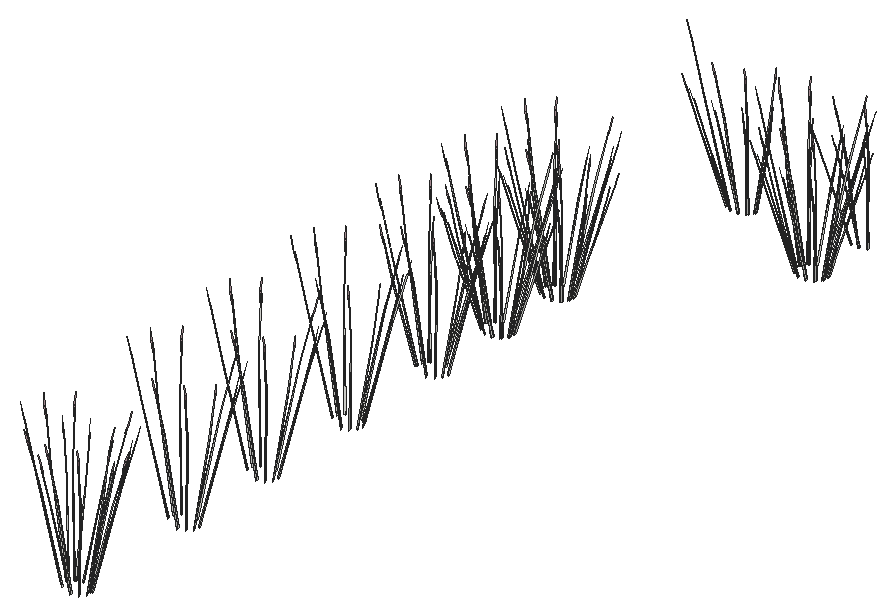
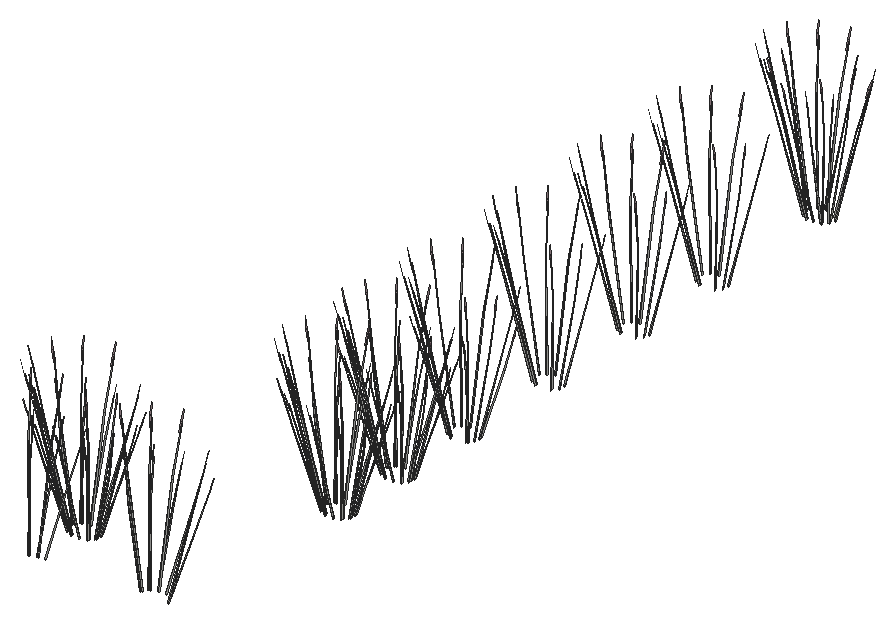
# SketchUp Ruby script. Lengths in inches.
U = 1.inch
M = Sketchup.active_model
def pt(a) = Geom::Point3d.new(a.map { |v| v * U })
def face(e, loops, mat)
  f = e.add_face(loops[0].map { |a| pt(a) })
  loops[1..].each { |l| e.add_face(l.map { |a| pt(a) }).erase! }
  f.material = f.back_material = mat if mat
  f
end
# faces: each face lists its corners as indices into pts; further lists are holes
def faces(e, pts, list, mat = nil) = list.each { |f| face(e, (f[0].is_a?(Array) ? f : [f]).map { |l| l.map { |i| pts[i] } }, mat) }
# xy, xz, yz: faces in a plane at the given z, y or x. An outline is a flat list of corners, or four numbers for a rectangle; further outlines are holes
def ring(l) = l.size == 4 ? [[l[0], l[1]], [l[2], l[1]], [l[2], l[3]], [l[0], l[3]]] : l.each_slice(2).to_a
def flat(e, list, mat, &to3) = list.each { |f| face(e, (f[0].is_a?(Array) ? f : [f]).map { |l| ring(l).map { |u, v| to3.(u, v) } }, mat) }
def xy(e, z, list, mat = nil) = flat(e, list, mat) { |x, y| [x, y, z] }
def xz(e, y, list, mat = nil) = flat(e, list, mat) { |x, z| [x, y, z] }
def yz(e, x, list, mat = nil) = flat(e, list, mat) { |y, z| [x, y, z] }
def lines(e, pts, list) = list.each { |a, b| e.add_line(pt(pts[a]), pt(pts[b])) }
# prism: a flat outline (further loops are holes) pulled along v
def prism(e, loops, v, mat = nil)
  f = face(e, loops, mat); d = Geom::Vector3d.new(v.map { |x| x * U })
  f.pushpull(f.normal.samedirection?(d) ? d.length : -d.length)
end
def box(e, o, s, mat = nil) = prism(e, [[o, [o[0] + s[0], o[1], o[2]], [o[0] + s[0], o[1] + s[1], o[2]], [o[0], o[1] + s[1], o[2]]]], [0, 0, s[2]], mat)
def at(x, y, z, deg = 0) = Geom::Transformation.translation(pt([x, y, z])) * Geom::Transformation.rotation(ORIGIN, Z_AXIS, deg.degrees)
def axes(o, x, y, z) = Geom::Transformation.new([*x, 0, *y, 0, *z, 0, *pt(o).to_a, 1])
def part(name) = M.definitions.add(name)
# library, detail: a bought-in or finely detailed component or shape, given as its bounding box
def library(name, o, s) = part(name).tap { |d| box(d.entities, o, s) }
def detail(e, o, s) = box(e.add_group.entities, o, s)
def put(e, d, t, mat = nil) = e.add_instance(d, t).tap { |i| i.material = mat if mat }
def group(e, t, mat = nil) = e.add_group.tap { |g| g.transformation = t; g.material = mat if mat }.entities
root = M.entities
M.materials.add("LightPink_Translucent").color = [144, 107, 117]
M.materials["LightPink_Translucent"].alpha = 0.75
c1 = part("blade")
p = [[2.15,0.21,22],[0,0.17,0],[0.09,0.45,0],[2.18,0.31,22],[2.29,0.31,22],[0.38,0.45,0],
  [2.48,0.24,33],[2.49,0.24,33],[2.48,0.22,33]]
faces(c1.entities,p,[[0,1,2,3],[4,5,2,3],[6,3,4,7],[8,0,3,6]])
c2 = part("seeds")
p = [[0.3,-0.1,1.38],[-0.01,-0.03,1.59],[-0.01,-0.03,0.03],[0.14,-0.07,-0.07],[0.29,-0.03,3],[0.15,0.01,3.11]]
faces(c2.entities,p,[[0,1,2,3],[1,0,4,5]],"LightPink_Translucent")
c3 = part("blade with seeds")
put(c3.entities,c1,at(0,0,0))
put(c3.entities,c2,axes([2.4,0.25,30.99],[1.5799,-0.05474,1.17369],[-0.12525,1.92788,0.29478],[-0.07173,-0.02425,1.56792]))
put(root,c3,axes([672.23,166.16,513.93],[0.64106,0.14927,0.39842],[-0.21921,0.49074,0.32852],[-0.03852,-0.19299,0.82444]))
put(root,c3,axes([672.22,166.52,514.19],[-0.19614,0.43908,0.29394],[-0.57222,-0.12807,-0.37948],[-0.05247,-0.17678,0.72609]))
put(root,c3,axes([673.68,166.71,513.93],[0.46327,0.38957,0.39842],[-0.49199,0.33598,0.32852],[0.08546,-0.18277,0.82444]))
put(root,c3,axes([674.61,167.77,513.93],[0.16135,0.52549,0.39842],[-0.63294,0.0912,0.32852],[0.18654,-0.12359,0.82444]))
put(root,c3,axes([669.7,167.22,514.19],[0.37017,0.35748,0.29394],[-0.42268,0.3384,-0.37948],[-0.21476,-0.05149,0.72609]))
put(root,c3,axes([674.31,169.0625,514.19],[-0.54068,-0.15928,0.29394],[0.1577,-0.46469,-0.37948],[0.21769,-0.04261,0.72609]))
put(root,c3,axes([668.65,168.21,513.93],[0.18381,-0.5206,0.39842],[0.60429,0.17802,0.32852],[-0.23764,0.03129,0.82444]))
put(root,c3,axes([674.75,169.07,513.93],[-0.18381,0.5206,0.39842],[-0.60429,-0.17802,0.32852],[0.23764,-0.03129,0.82444]))
put(root,c3,axes([673.7,170.07,514.19],[-0.37017,-0.35748,0.29394],[0.42268,-0.3384,-0.37948],[0.21476,0.05149,0.72609]))
put(root,c3,axes([668.8,169.51,513.93],[-0.16135,-0.52549,0.39842],[0.63294,-0.0912,0.32852],[-0.18654,0.12359,0.82444]))
put(root,c3,axes([669.18,169.34,514.19],[0.56631,-0.0816,0.29394],[0.14954,0.46647,-0.37948],[-0.16229,0.12529,0.72609]))
put(root,c3,axes([674.08,170.25,513.93],[-0.47971,0.37622,0.39842],[-0.41372,-0.39954,0.32852],[0.22506,0.0694,0.82444]))
put(root,c3,axes([669.95,170.26,514.19],[0.4402,-0.30062,0.29394],[0.41671,0.34326,-0.37948],[-0.0634,0.1744,0.72609]))
put(root,c3,axes([669.72,170.57,513.93],[-0.46327,-0.38957,0.39842],[0.49199,-0.33598,0.32852],[-0.08546,0.18277,0.82444]))
put(root,c3,axes([671.18,170.76,514.19],[0.19614,-0.43908,0.29394],[0.57222,0.12807,-0.37948],[0.05247,0.17678,0.72609]))
put(root,c3,axes([672.77,171,513.93],[-0.64708,0.13103,0.39842],[-0.1123,-0.514,0.32852],[0.15218,0.15149,0.82444]))
put(root,c3,axes([672.23,193.62,513.93],[0.64106,0.14927,0.39842],[-0.21921,0.49074,0.32852],[-0.03852,-0.19299,0.82444]))
put(root,c3,axes([673.68,194.17,513.93],[0.46327,0.38957,0.39842],[-0.49199,0.33598,0.32852],[0.08546,-0.18277,0.82444]))
put(root,c3,axes([674.61,195.23,513.93],[0.16135,0.52549,0.39842],[-0.63294,0.0912,0.32852],[0.18654,-0.12359,0.82444]))
put(root,c3,axes([668.65,195.67,513.93],[0.18381,-0.5206,0.39842],[0.60429,0.17802,0.32852],[-0.23764,0.03129,0.82444]))
put(root,c3,axes([674.75,196.53,513.93],[-0.18381,0.5206,0.39842],[-0.60429,-0.17802,0.32852],[0.23764,-0.03129,0.82444]))
put(root,c3,axes([668.8,196.97,513.93],[-0.16135,-0.52549,0.39842],[0.63294,-0.0912,0.32852],[-0.18654,0.12359,0.82444]))
put(root,c3,axes([674.08,197.71,513.93],[-0.47971,0.37622,0.39842],[-0.41372,-0.39954,0.32852],[0.22506,0.0694,0.82444]))
put(root,c3,axes([669.72,198.03,513.93],[-0.46327,-0.38957,0.39842],[0.49199,-0.33598,0.32852],[-0.08546,0.18277,0.82444]))
put(root,c3,axes([672.77,198.46,513.93],[-0.64708,0.13103,0.39842],[-0.1123,-0.514,0.32852],[0.15218,0.15149,0.82444]))
put(root,c3,axes([672.23,213.91,513.93],[0.64106,0.14927,0.39842],[-0.21921,0.49074,0.32852],[-0.03852,-0.19299,0.82444]))
put(root,c3,axes([673.68,214.46,513.93],[0.46327,0.38957,0.39842],[-0.49199,0.33598,0.32852],[0.08546,-0.18277,0.82444]))
put(root,c3,axes([674.61,215.52,513.93],[0.16135,0.52549,0.39842],[-0.63294,0.0912,0.32852],[0.18654,-0.12359,0.82444]))
put(root,c3,axes([668.65,215.96,513.93],[0.18381,-0.5206,0.39842],[0.60429,0.17802,0.32852],[-0.23764,0.03129,0.82444]))
put(root,c3,axes([674.75,216.82,513.93],[-0.18381,0.5206,0.39842],[-0.60429,-0.17802,0.32852],[0.23764,-0.03129,0.82444]))
put(root,c3,axes([668.8,217.26,513.93],[-0.16135,-0.52549,0.39842],[0.63294,-0.0912,0.32852],[-0.18654,0.12359,0.82444]))
put(root,c3,axes([674.08,218,513.93],[-0.47971,0.37622,0.39842],[-0.41372,-0.39954,0.32852],[0.22506,0.0694,0.82444]))
put(root,c3,axes([669.72,218.32,513.93],[-0.46327,-0.38957,0.39842],[0.49199,-0.33598,0.32852],[-0.08546,0.18277,0.82444]))
put(root,c3,axes([672.77,218.75,513.93],[-0.64708,0.13103,0.39842],[-0.1123,-0.514,0.32852],[0.15218,0.15149,0.82444]))
put(root,c3,axes([672.23,235.61,513.93],[0.64106,0.14927,0.39842],[-0.21921,0.49074,0.32852],[-0.03852,-0.19299,0.82444]))
put(root,c3,axes([673.68,236.16,513.93],[0.46327,0.38957,0.39842],[-0.49199,0.33598,0.32852],[0.08546,-0.18277,0.82444]))
put(root,c3,axes([674.61,237.22,513.93],[0.16135,0.52549,0.39842],[-0.63294,0.0912,0.32852],[0.18654,-0.12359,0.82444]))
put(root,c3,axes([668.65,237.66,513.93],[0.18381,-0.5206,0.39842],[0.60429,0.17802,0.32852],[-0.23764,0.03129,0.82444]))
put(root,c3,axes([674.75,238.52,513.93],[-0.18381,0.5206,0.39842],[-0.60429,-0.17802,0.32852],[0.23764,-0.03129,0.82444]))
put(root,c3,axes([668.8,238.96,513.93],[-0.16135,-0.52549,0.39842],[0.63294,-0.0912,0.32852],[-0.18654,0.12359,0.82444]))
put(root,c3,axes([674.08,239.7,513.93],[-0.47971,0.37622,0.39842],[-0.41372,-0.39954,0.32852],[0.22506,0.0694,0.82444]))
put(root,c3,axes([669.72,240.02,513.93],[-0.46327,-0.38957,0.39842],[0.49199,-0.33598,0.32852],[-0.08546,0.18277,0.82444]))
put(root,c3,axes([672.77,240.45,513.93],[-0.64708,0.13103,0.39842],[-0.1123,-0.514,0.32852],[0.15218,0.15149,0.82444]))
put(root,c3,axes([672.23,257.45,513.93],[0.64106,0.14927,0.39842],[-0.21921,0.49074,0.32852],[-0.03852,-0.19299,0.82444]))
put(root,c3,axes([673.68,258,513.93],[0.46327,0.38957,0.39842],[-0.49199,0.33598,0.32852],[0.08546,-0.18277,0.82444]))
put(root,c3,axes([674.61,259.0625,513.93],[0.16135,0.52549,0.39842],[-0.63294,0.0912,0.32852],[0.18654,-0.12359,0.82444]))
put(root,c3,axes([668.65,259.51,513.93],[0.18381,-0.5206,0.39842],[0.60429,0.17802,0.32852],[-0.23764,0.03129,0.82444]))
put(root,c3,axes([668.6,259.37,513.93],[-0.23895,-0.38931,0.05337],[0.43573,-0.19055,0.42015],[-0.19208,0.0376,0.64067]))
put(root,c3,axes([674.75,260.36,513.93],[-0.18381,0.5206,0.39842],[-0.60429,-0.17802,0.32852],[0.23764,-0.03129,0.82444]))
put(root,c3,axes([668.8,260.8,513.93],[-0.16135,-0.52549,0.39842],[0.63294,-0.0912,0.32852],[-0.18654,0.12359,0.82444]))
put(root,c3,axes([674.08,261.54,513.93],[-0.47971,0.37622,0.39842],[-0.41372,-0.39954,0.32852],[0.22506,0.0694,0.82444]))
put(root,c3,axes([669.55,261.83,513.93],[-0.53464,-0.0266,0.05337],[0.01466,-0.40172,0.42015],[-0.05594,0.15388,0.64067]))
put(root,c3,axes([669.72,261.87,513.93],[-0.46327,-0.38957,0.39842],[0.49199,-0.33598,0.32852],[-0.08546,0.18277,0.82444]))
put(root,c3,axes([672.65,262.4,513.93],[-0.29569,0.36271,0.05337],[-0.42107,-0.21117,0.42015],[0.13613,0.11629,0.64067]))
put(root,c3,axes([672.77,262.29,513.93],[-0.64708,0.13103,0.39842],[-0.1123,-0.514,0.32852],[0.15218,0.15149,0.82444]))
put(root,c3,axes([672.23,274.3125,513.93],[0.64106,0.14927,0.39842],[-0.21921,0.49074,0.32852],[-0.03852,-0.19299,0.82444]))
put(root,c3,axes([672.4,274.28,513.93],[0.47939,-0.19405,0.05337],[0.23464,0.35385,0.42015],[-0.0463,-0.15598,0.64067]))
put(root,c3,axes([670.76,274.33,513.93],[0.29569,-0.36271,0.05337],[0.42107,0.21117,0.42015],[-0.13613,-0.11629,0.64067]))
put(root,c3,axes([673.68,274.86,513.93],[0.46327,0.38957,0.39842],[-0.49199,0.33598,0.32852],[0.08546,-0.18277,0.82444]))
put(root,c3,axes([673.85,274.9,513.93],[0.53464,0.0266,0.05337],[-0.01466,0.40172,0.42015],[0.05594,-0.15388,0.64067]))
put(root,c3,axes([669.37,275.04,513.93],[0.03276,-0.43418,0.05337],[0.49468,0.0119,0.42015],[-0.18949,-0.04543,0.64067]))
put(root,c3,axes([674.73,276.02,513.93],[0.44663,0.24013,0.05337],[-0.26003,0.34195,0.42015],[0.14319,-0.11055,0.64067]))
put(root,c3,axes([674.61,275.92,513.93],[0.16135,0.52549,0.39842],[-0.63294,0.0912,0.32852],[0.18654,-0.12359,0.82444]))
put(root,c3,axes([668.65,276.36,513.93],[0.18381,-0.5206,0.39842],[0.60429,0.17802,0.32852],[-0.23764,0.03129,0.82444]))
put(root,c3,axes([668.6,276.23,513.93],[-0.23895,-0.38931,0.05337],[0.43573,-0.19055,0.42015],[-0.19208,0.0376,0.64067]))
put(root,c3,axes([674.8,277.36,513.93],[0.23895,0.38931,0.05337],[-0.43573,0.19055,0.42015],[0.19208,-0.0376,0.64067]))
put(root,c3,axes([674.75,277.22,513.93],[-0.18381,0.5206,0.39842],[-0.60429,-0.17802,0.32852],[0.23764,-0.03129,0.82444]))
put(root,c3,axes([668.8,277.66,513.93],[-0.16135,-0.52549,0.39842],[0.63294,-0.0912,0.32852],[-0.18654,0.12359,0.82444]))
put(root,c3,axes([668.67,277.5625,513.93],[-0.44663,-0.24013,0.05337],[0.26003,-0.34195,0.42015],[-0.14319,0.11055,0.64067]))
put(root,c3,axes([674.04,278.54,513.93],[-0.03276,0.43418,0.05337],[-0.49468,-0.0119,0.42015],[0.18949,0.04543,0.64067]))
put(root,c3,axes([674.08,278.4,513.93],[-0.47971,0.37622,0.39842],[-0.41372,-0.39954,0.32852],[0.22506,0.0694,0.82444]))
put(root,c3,axes([669.55,278.6875,513.93],[-0.53464,-0.0266,0.05337],[0.01466,-0.40172,0.42015],[-0.05594,0.15388,0.64067]))
put(root,c3,axes([669.72,278.73,513.93],[-0.46327,-0.38957,0.39842],[0.49199,-0.33598,0.32852],[-0.08546,0.18277,0.82444]))
put(root,c3,axes([672.65,279.25,513.93],[-0.29569,0.36271,0.05337],[-0.42107,-0.21117,0.42015],[0.13613,0.11629,0.64067]))
put(root,c3,axes([672.77,279.15,513.93],[-0.64708,0.13103,0.39842],[-0.1123,-0.514,0.32852],[0.15218,0.15149,0.82444]))
put(root,c3,axes([671,279.31,513.93],[-0.47939,0.19405,0.05337],[-0.23464,-0.35385,0.42015],[0.0463,0.15598,0.64067]))
put(root,c3,axes([672.23,289.65,513.93],[0.64106,0.14927,0.39842],[-0.21921,0.49074,0.32852],[-0.03852,-0.19299,0.82444]))
put(root,c3,axes([672.4,289.61,513.93],[0.47939,-0.19405,0.05337],[0.23464,0.35385,0.42015],[-0.0463,-0.15598,0.64067]))
put(root,c3,axes([670.76,289.67,513.93],[0.29569,-0.36271,0.05337],[0.42107,0.21117,0.42015],[-0.13613,-0.11629,0.64067]))
put(root,c3,axes([673.68,290.19,513.93],[0.46327,0.38957,0.39842],[-0.49199,0.33598,0.32852],[0.08546,-0.18277,0.82444]))
put(root,c3,axes([673.85,290.23,513.93],[0.53464,0.0266,0.05337],[-0.01466,0.40172,0.42015],[0.05594,-0.15388,0.64067]))
put(root,c3,axes([669.37,290.38,513.93],[0.03276,-0.43418,0.05337],[0.49468,0.0119,0.42015],[-0.18949,-0.04543,0.64067]))
put(root,c3,axes([674.73,291.36,513.93],[0.44663,0.24013,0.05337],[-0.26003,0.34195,0.42015],[0.14319,-0.11055,0.64067]))
put(root,c3,axes([674.61,291.26,513.93],[0.16135,0.52549,0.39842],[-0.63294,0.0912,0.32852],[0.18654,-0.12359,0.82444]))
put(root,c3,axes([668.65,291.7,513.93],[0.18381,-0.5206,0.39842],[0.60429,0.17802,0.32852],[-0.23764,0.03129,0.82444]))
put(root,c3,axes([668.6,291.5625,513.93],[-0.23895,-0.38931,0.05337],[0.43573,-0.19055,0.42015],[-0.19208,0.0376,0.64067]))
put(root,c3,axes([674.8,292.69,513.93],[0.23895,0.38931,0.05337],[-0.43573,0.19055,0.42015],[0.19208,-0.0376,0.64067]))
put(root,c3,axes([674.75,292.55,513.93],[-0.18381,0.5206,0.39842],[-0.60429,-0.17802,0.32852],[0.23764,-0.03129,0.82444]))
put(root,c3,axes([668.8,293,513.93],[-0.16135,-0.52549,0.39842],[0.63294,-0.0912,0.32852],[-0.18654,0.12359,0.82444]))
put(root,c3,axes([668.67,292.89,513.93],[-0.44663,-0.24013,0.05337],[0.26003,-0.34195,0.42015],[-0.14319,0.11055,0.64067]))
put(root,c3,axes([674.04,293.875,513.93],[-0.03276,0.43418,0.05337],[-0.49468,-0.0119,0.42015],[0.18949,0.04543,0.64067]))
put(root,c3,axes([674.08,293.74,513.93],[-0.47971,0.37622,0.39842],[-0.41372,-0.39954,0.32852],[0.22506,0.0694,0.82444]))
put(root,c3,axes([669.55,294.02,513.93],[-0.53464,-0.0266,0.05337],[0.01466,-0.40172,0.42015],[-0.05594,0.15388,0.64067]))
put(root,c3,axes([669.72,294.06,513.93],[-0.46327,-0.38957,0.39842],[0.49199,-0.33598,0.32852],[-0.08546,0.18277,0.82444]))
put(root,c3,axes([672.65,294.59,513.93],[-0.29569,0.36271,0.05337],[-0.42107,-0.21117,0.42015],[0.13613,0.11629,0.64067]))
put(root,c3,axes([672.77,294.49,513.93],[-0.64708,0.13103,0.39842],[-0.1123,-0.514,0.32852],[0.15218,0.15149,0.82444]))
put(root,c3,axes([671,294.64,513.93],[-0.47939,0.19405,0.05337],[-0.23464,-0.35385,0.42015],[0.0463,0.15598,0.64067]))
put(root,c3,axes([699.83,320.34,513.93],[0.64106,0.14927,0.39842],[-0.21921,0.49074,0.32852],[-0.03852,-0.19299,0.82444]))
put(root,c3,axes([700,320.3,513.93],[0.47939,-0.19405,0.05337],[0.23464,0.35385,0.42015],[-0.0463,-0.15598,0.64067]))
put(root,c3,axes([698.36,320.36,513.93],[0.29569,-0.36271,0.05337],[0.42107,0.21117,0.42015],[-0.13613,-0.11629,0.64067]))
put(root,c3,axes([701.29,320.89,513.93],[0.46327,0.38957,0.39842],[-0.49199,0.33598,0.32852],[0.08546,-0.18277,0.82444]))
put(root,c3,axes([701.46,320.92,513.93],[0.53464,0.0266,0.05337],[-0.01466,0.40172,0.42015],[0.05594,-0.15388,0.64067]))
put(root,c3,axes([696.97,321.07,513.93],[0.03276,-0.43418,0.05337],[0.49468,0.0119,0.42015],[-0.18949,-0.04543,0.64067]))
put(root,c3,axes([702.34,322.05,513.93],[0.44663,0.24013,0.05337],[-0.26003,0.34195,0.42015],[0.14319,-0.11055,0.64067]))
put(root,c3,axes([702.21,321.95,513.93],[0.16135,0.52549,0.39842],[-0.63294,0.0912,0.32852],[0.18654,-0.12359,0.82444]))
put(root,c3,axes([696.25,322.39,513.93],[0.18381,-0.5206,0.39842],[0.60429,0.17802,0.32852],[-0.23764,0.03129,0.82444]))
put(root,c3,axes([696.21,322.25,513.93],[-0.23895,-0.38931,0.05337],[0.43573,-0.19055,0.42015],[-0.19208,0.0376,0.64067]))
put(root,c3,axes([702.41,323.38,513.93],[0.23895,0.38931,0.05337],[-0.43573,0.19055,0.42015],[0.19208,-0.0376,0.64067]))
put(root,c3,axes([702.36,323.25,513.93],[-0.18381,0.5206,0.39842],[-0.60429,-0.17802,0.32852],[0.23764,-0.03129,0.82444]))
put(root,c3,axes([696.4,323.6875,513.93],[-0.16135,-0.52549,0.39842],[0.63294,-0.0912,0.32852],[-0.18654,0.12359,0.82444]))
put(root,c3,axes([696.28,323.59,513.93],[-0.44663,-0.24013,0.05337],[0.26003,-0.34195,0.42015],[-0.14319,0.11055,0.64067]))
put(root,c3,axes([701.64,324.57,513.93],[-0.03276,0.43418,0.05337],[-0.49468,-0.0119,0.42015],[0.18949,0.04543,0.64067]))
put(root,c3,axes([701.6875,324.43,513.93],[-0.47971,0.37622,0.39842],[-0.41372,-0.39954,0.32852],[0.22506,0.0694,0.82444]))
put(root,c3,axes([697.15,324.71,513.93],[-0.53464,-0.0266,0.05337],[0.01466,-0.40172,0.42015],[-0.05594,0.15388,0.64067]))
put(root,c3,axes([677.67,330.5625,513.93],[0.64106,0.14927,0.39842],[-0.21921,0.49074,0.32852],[-0.03852,-0.19299,0.82444]))
put(root,c3,axes([697.32,324.75,513.93],[-0.46327,-0.38957,0.39842],[0.49199,-0.33598,0.32852],[-0.08546,0.18277,0.82444]))
put(root,c3,axes([677.84,330.53,513.93],[0.47939,-0.19405,0.05337],[0.23464,0.35385,0.42015],[-0.0463,-0.15598,0.64067]))
put(root,c3,axes([700.25,325.28,513.93],[-0.29569,0.36271,0.05337],[-0.42107,-0.21117,0.42015],[0.13613,0.11629,0.64067]))
put(root,c3,axes([676.2,330.58,513.93],[0.29569,-0.36271,0.05337],[0.42107,0.21117,0.42015],[-0.13613,-0.11629,0.64067]))
put(root,c3,axes([700.375,325.18,513.93],[-0.64708,0.13103,0.39842],[-0.1123,-0.514,0.32852],[0.15218,0.15149,0.82444]))
put(root,c3,axes([698.61,325.33,513.93],[-0.47939,0.19405,0.05337],[-0.23464,-0.35385,0.42015],[0.0463,0.15598,0.64067]))
put(root,c3,axes([679.13,331.11,513.93],[0.46327,0.38957,0.39842],[-0.49199,0.33598,0.32852],[0.08546,-0.18277,0.82444]))
put(root,c3,axes([679.3,331.15,513.93],[0.53464,0.0266,0.05337],[-0.01466,0.40172,0.42015],[0.05594,-0.15388,0.64067]))
put(root,c3,axes([674.8125,331.29,513.93],[0.03276,-0.43418,0.05337],[0.49468,0.0119,0.42015],[-0.18949,-0.04543,0.64067]))
put(root,c3,axes([699.83,333.84,513.93],[0.64106,0.14927,0.39842],[-0.21921,0.49074,0.32852],[-0.03852,-0.19299,0.82444]))
put(root,c3,axes([680.18,332.27,513.93],[0.44663,0.24013,0.05337],[-0.26003,0.34195,0.42015],[0.14319,-0.11055,0.64067]))
put(root,c3,axes([680.05,332.17,513.93],[0.16135,0.52549,0.39842],[-0.63294,0.0912,0.32852],[0.18654,-0.12359,0.82444]))
put(root,c3,axes([700,333.8,513.93],[0.47939,-0.19405,0.05337],[0.23464,0.35385,0.42015],[-0.0463,-0.15598,0.64067]))
put(root,c3,axes([698.36,333.86,513.93],[0.29569,-0.36271,0.05337],[0.42107,0.21117,0.42015],[-0.13613,-0.11629,0.64067]))
put(root,c3,axes([701.29,334.39,513.93],[0.46327,0.38957,0.39842],[-0.49199,0.33598,0.32852],[0.08546,-0.18277,0.82444]))
put(root,c3,axes([701.46,334.42,513.93],[0.53464,0.0266,0.05337],[-0.01466,0.40172,0.42015],[0.05594,-0.15388,0.64067]))
put(root,c3,axes([674.09,332.61,513.93],[0.18381,-0.5206,0.39842],[0.60429,0.17802,0.32852],[-0.23764,0.03129,0.82444]))
